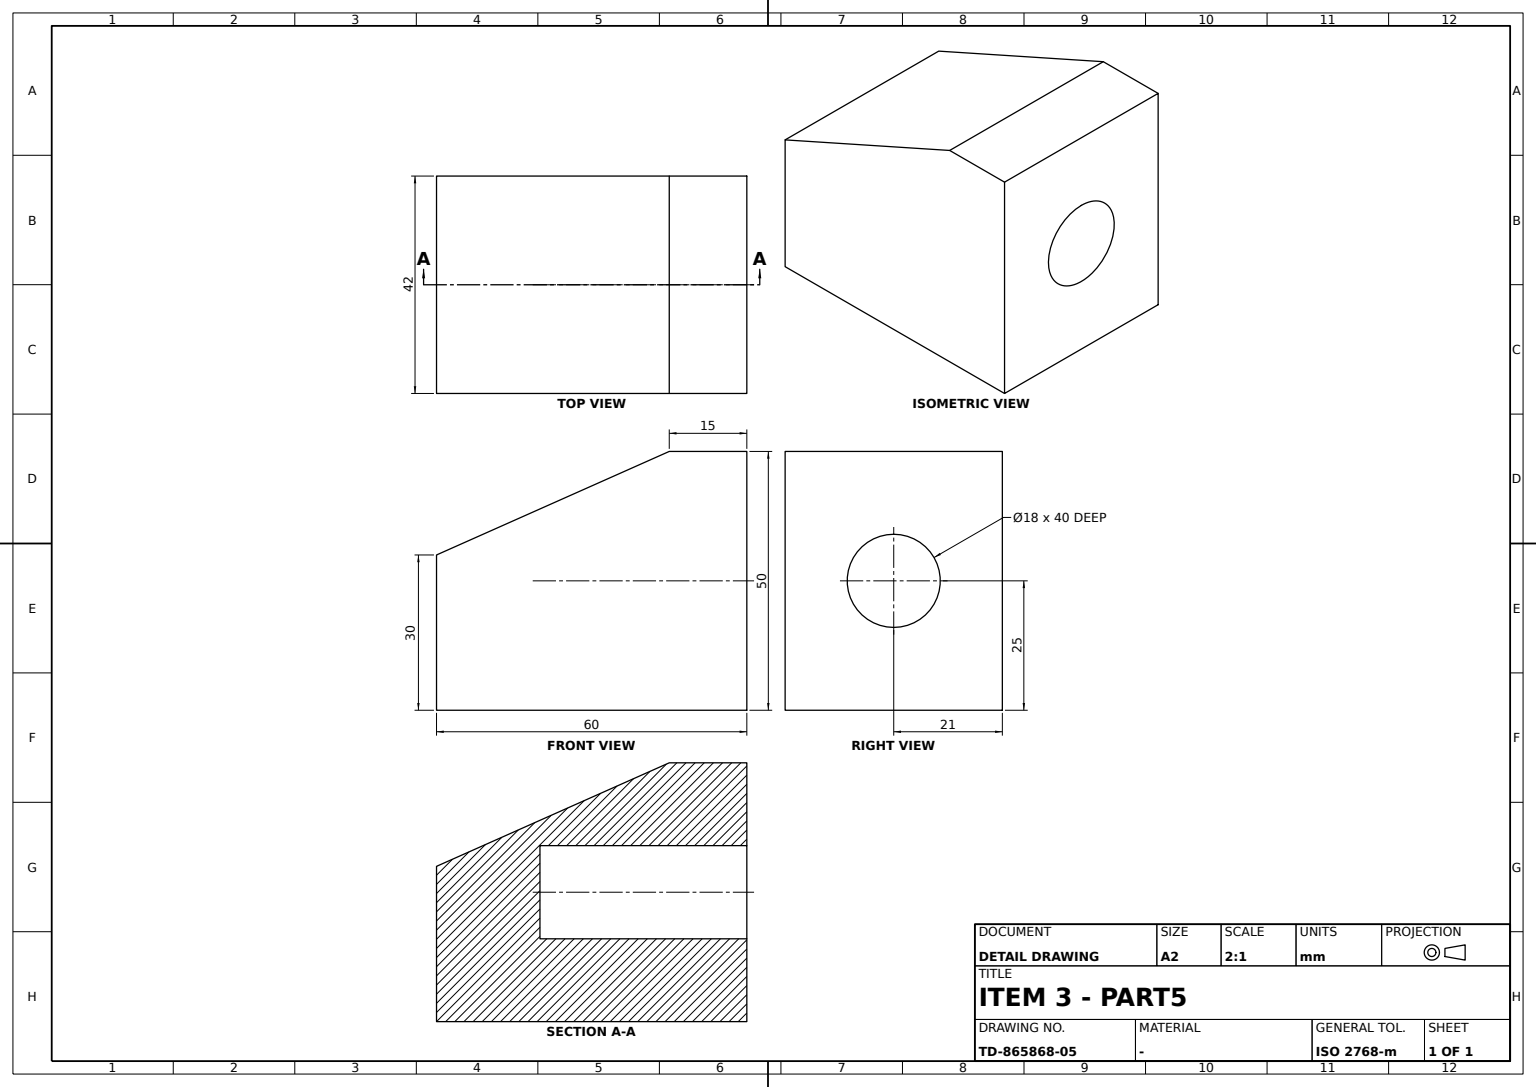
ISO-10303-21;
HEADER;
FILE_DESCRIPTION((''),'2;1');
FILE_NAME('','',(''),(''),'','','');
FILE_SCHEMA(('AUTOMOTIVE_DESIGN'));
ENDSEC;
DATA;
#1=APPLICATION_CONTEXT('');
#2=PRODUCT_CONTEXT('',#1,'mechanical');
#3=PRODUCT('','','',(#2));
#4=PRODUCT_DEFINITION_FORMATION('','',#3);
#5=PRODUCT_DEFINITION_CONTEXT('',#1,'design');
#6=PRODUCT_DEFINITION('','',#4,#5);
#7=PRODUCT_DEFINITION_SHAPE('','',#6);
#8=(LENGTH_UNIT()NAMED_UNIT(*)SI_UNIT(.MILLI.,.METRE.));
#9=(NAMED_UNIT(*)PLANE_ANGLE_UNIT()SI_UNIT($,.RADIAN.));
#10=(NAMED_UNIT(*)SI_UNIT($,.STERADIAN.)SOLID_ANGLE_UNIT());
#11=UNCERTAINTY_MEASURE_WITH_UNIT(LENGTH_MEASURE(0.005),#8,'distance_accuracy_value','');
#12=(GEOMETRIC_REPRESENTATION_CONTEXT(3)GLOBAL_UNCERTAINTY_ASSIGNED_CONTEXT((#11))GLOBAL_UNIT_ASSIGNED_CONTEXT((#8,#9,#10))REPRESENTATION_CONTEXT('',''));
#13=CARTESIAN_POINT('',(0.,60.,34.));
#14=VERTEX_POINT('',#13);
#15=CARTESIAN_POINT('',(0.,60.,25.));
#16=DIRECTION('',(0.,1.,0.));
#17=DIRECTION('',(0.,0.,1.));
#18=AXIS2_PLACEMENT_3D('',#15,#16,#17);
#19=CIRCLE('',#18,9.);
#20=EDGE_CURVE('',#14,#14,#19,.T.);
#21=ORIENTED_EDGE('',*,*,#20,.F.);
#22=EDGE_LOOP('',(#21));
#23=FACE_BOUND('',#22,.T.);
#24=CARTESIAN_POINT('',(-21.,60.,50.));
#25=VERTEX_POINT('',#24);
#26=CARTESIAN_POINT('',(21.,60.,50.));
#27=VERTEX_POINT('',#26);
#28=CARTESIAN_POINT('',(0.,60.,50.));
#29=DIRECTION('',(1.,0.,0.));
#30=VECTOR('',#29,1000.);
#31=LINE('',#28,#30);
#32=EDGE_CURVE('',#25,#27,#31,.T.);
#33=ORIENTED_EDGE('',*,*,#32,.T.);
#34=CARTESIAN_POINT('',(21.,60.,0.));
#35=VERTEX_POINT('',#34);
#36=VECTOR('',#17,1000.);
#37=LINE('',#34,#36);
#38=EDGE_CURVE('',#35,#27,#37,.T.);
#39=ORIENTED_EDGE('',*,*,#38,.F.);
#40=CARTESIAN_POINT('',(-21.,60.,0.));
#41=VERTEX_POINT('',#40);
#42=CARTESIAN_POINT('',(0.,60.,0.));
#43=LINE('',#42,#30);
#44=EDGE_CURVE('',#41,#35,#43,.T.);
#45=ORIENTED_EDGE('',*,*,#44,.F.);
#46=LINE('',#40,#36);
#47=EDGE_CURVE('',#41,#25,#46,.T.);
#48=ORIENTED_EDGE('',*,*,#47,.T.);
#49=EDGE_LOOP('',(#33,#39,#45,#48));
#50=FACE_BOUND('',#49,.T.);
#51=AXIS2_PLACEMENT_3D('',#42,#16,#17);
#52=PLANE('',#51);
#53=ADVANCED_FACE('',(#23,#50),#52,.T.);
#54=ORIENTED_EDGE('',*,*,#47,.F.);
#55=CARTESIAN_POINT('',(-21.,0.,0.));
#56=VERTEX_POINT('',#55);
#57=VECTOR('',#16,1000.);
#58=LINE('',#55,#57);
#59=EDGE_CURVE('',#56,#41,#58,.T.);
#60=ORIENTED_EDGE('',*,*,#59,.F.);
#61=CARTESIAN_POINT('',(-21.,0.,30.));
#62=VERTEX_POINT('',#61);
#63=DIRECTION('',(0.,0.,-1.));
#64=VECTOR('',#63,1000.);
#65=LINE('',#55,#64);
#66=EDGE_CURVE('',#62,#56,#65,.T.);
#67=ORIENTED_EDGE('',*,*,#66,.F.);
#68=CARTESIAN_POINT('',(-21.,45.,50.));
#69=VERTEX_POINT('',#68);
#70=CARTESIAN_POINT('',(-21.,-11.134021,25.051546));
#71=DIRECTION('',(0.,-0.913811549,-0.406138466));
#72=VECTOR('',#71,1000.);
#73=LINE('',#70,#72);
#74=EDGE_CURVE('',#69,#62,#73,.T.);
#75=ORIENTED_EDGE('',*,*,#74,.F.);
#76=CARTESIAN_POINT('',(-21.,0.,50.));
#77=DIRECTION('',(0.,-1.,0.));
#78=VECTOR('',#77,1000.);
#79=LINE('',#76,#78);
#80=EDGE_CURVE('',#25,#69,#79,.T.);
#81=ORIENTED_EDGE('',*,*,#80,.F.);
#82=EDGE_LOOP('',(#54,#60,#67,#75,#81));
#83=FACE_BOUND('',#82,.T.);
#84=AXIS2_PLACEMENT_3D('',#55,#29,#16);
#85=PLANE('',#84);
#86=ADVANCED_FACE('',(#83),#85,.F.);
#87=CARTESIAN_POINT('',(21.,0.,30.));
#88=VERTEX_POINT('',#87);
#89=CARTESIAN_POINT('',(0.,0.,30.));
#90=LINE('',#89,#30);
#91=EDGE_CURVE('',#62,#88,#90,.T.);
#92=ORIENTED_EDGE('',*,*,#91,.F.);
#93=ORIENTED_EDGE('',*,*,#66,.T.);
#94=CARTESIAN_POINT('',(21.,0.,0.));
#95=VERTEX_POINT('',#94);
#96=CARTESIAN_POINT('',(0.,0.,0.));
#97=LINE('',#96,#30);
#98=EDGE_CURVE('',#56,#95,#97,.T.);
#99=ORIENTED_EDGE('',*,*,#98,.T.);
#100=LINE('',#94,#64);
#101=EDGE_CURVE('',#88,#95,#100,.T.);
#102=ORIENTED_EDGE('',*,*,#101,.F.);
#103=EDGE_LOOP('',(#92,#93,#99,#102));
#104=FACE_BOUND('',#103,.T.);
#105=AXIS2_PLACEMENT_3D('',#89,#77,#63);
#106=PLANE('',#105);
#107=ADVANCED_FACE('',(#104),#106,.T.);
#108=ORIENTED_EDGE('',*,*,#20,.T.);
#109=EDGE_LOOP('',(#108));
#110=FACE_BOUND('',#109,.T.);
#111=CARTESIAN_POINT('',(0.,20.,34.));
#112=VERTEX_POINT('',#111);
#113=CARTESIAN_POINT('',(0.,20.,25.));
#114=AXIS2_PLACEMENT_3D('',#113,#16,#17);
#115=CIRCLE('',#114,9.);
#116=EDGE_CURVE('',#112,#112,#115,.T.);
#117=ORIENTED_EDGE('',*,*,#116,.F.);
#118=EDGE_LOOP('',(#117));
#119=FACE_BOUND('',#118,.T.);
#120=CARTESIAN_POINT('',(0.,40.,25.));
#121=DIRECTION('',(-1.,0.,0.));
#122=AXIS2_PLACEMENT_3D('',#120,#16,#121);
#123=CYLINDRICAL_SURFACE('',#122,9.);
#124=ADVANCED_FACE('',(#110,#119),#123,.F.);
#125=LINE('',#94,#57);
#126=EDGE_CURVE('',#95,#35,#125,.T.);
#127=ORIENTED_EDGE('',*,*,#126,.F.);
#128=ORIENTED_EDGE('',*,*,#98,.F.);
#129=ORIENTED_EDGE('',*,*,#59,.T.);
#130=ORIENTED_EDGE('',*,*,#44,.T.);
#131=EDGE_LOOP('',(#127,#128,#129,#130));
#132=FACE_BOUND('',#131,.T.);
#133=AXIS2_PLACEMENT_3D('',#96,#63,#16);
#134=PLANE('',#133);
#135=ADVANCED_FACE('',(#132),#134,.T.);
#136=ORIENTED_EDGE('',*,*,#116,.T.);
#137=EDGE_LOOP('',(#136));
#138=FACE_BOUND('',#137,.T.);
#139=CARTESIAN_POINT('',(0.,20.,0.));
#140=AXIS2_PLACEMENT_3D('',#139,#16,#121);
#141=PLANE('',#140);
#142=ADVANCED_FACE('',(#138),#141,.T.);
#143=ORIENTED_EDGE('',*,*,#74,.T.);
#144=ORIENTED_EDGE('',*,*,#91,.T.);
#145=CARTESIAN_POINT('',(21.,45.,50.));
#146=VERTEX_POINT('',#145);
#147=CARTESIAN_POINT('',(21.,-11.134021,25.051546));
#148=LINE('',#147,#72);
#149=EDGE_CURVE('',#146,#88,#148,.T.);
#150=ORIENTED_EDGE('',*,*,#149,.F.);
#151=CARTESIAN_POINT('',(0.,45.,50.));
#152=LINE('',#151,#30);
#153=EDGE_CURVE('',#69,#146,#152,.T.);
#154=ORIENTED_EDGE('',*,*,#153,.F.);
#155=EDGE_LOOP('',(#143,#144,#150,#154));
#156=FACE_BOUND('',#155,.T.);
#157=DIRECTION('',(0.,-0.406138466,0.913811549));
#158=AXIS2_PLACEMENT_3D('',#151,#157,#71);
#159=PLANE('',#158);
#160=ADVANCED_FACE('',(#156),#159,.T.);
#161=ORIENTED_EDGE('',*,*,#101,.T.);
#162=ORIENTED_EDGE('',*,*,#126,.T.);
#163=ORIENTED_EDGE('',*,*,#38,.T.);
#164=CARTESIAN_POINT('',(21.,0.,50.));
#165=LINE('',#164,#78);
#166=EDGE_CURVE('',#27,#146,#165,.T.);
#167=ORIENTED_EDGE('',*,*,#166,.T.);
#168=ORIENTED_EDGE('',*,*,#149,.T.);
#169=EDGE_LOOP('',(#161,#162,#163,#167,#168));
#170=FACE_BOUND('',#169,.T.);
#171=AXIS2_PLACEMENT_3D('',#94,#29,#16);
#172=PLANE('',#171);
#173=ADVANCED_FACE('',(#170),#172,.T.);
#174=ORIENTED_EDGE('',*,*,#153,.T.);
#175=ORIENTED_EDGE('',*,*,#166,.F.);
#176=ORIENTED_EDGE('',*,*,#32,.F.);
#177=ORIENTED_EDGE('',*,*,#80,.T.);
#178=EDGE_LOOP('',(#174,#175,#176,#177));
#179=FACE_BOUND('',#178,.T.);
#180=AXIS2_PLACEMENT_3D('',#28,#17,#77);
#181=PLANE('',#180);
#182=ADVANCED_FACE('',(#179),#181,.T.);
#183=CLOSED_SHELL('',(#53,#86,#107,#124,#135,#142,#160,#173,#182));
#184=MANIFOLD_SOLID_BREP('',#183);
#185=ADVANCED_BREP_SHAPE_REPRESENTATION('',(#184),#12);
#186=SHAPE_DEFINITION_REPRESENTATION(#7,#185);
ENDSEC;
END-ISO-10303-21;
